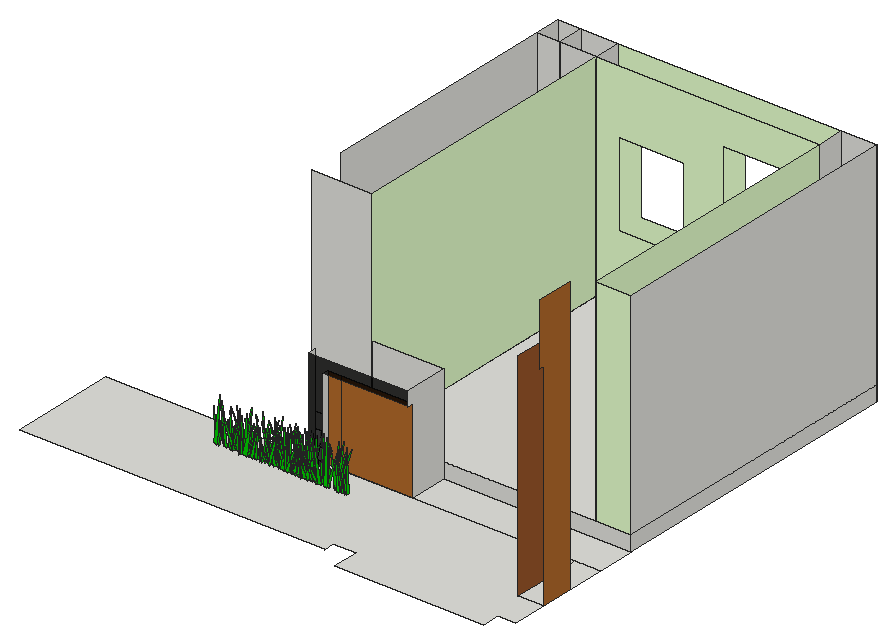
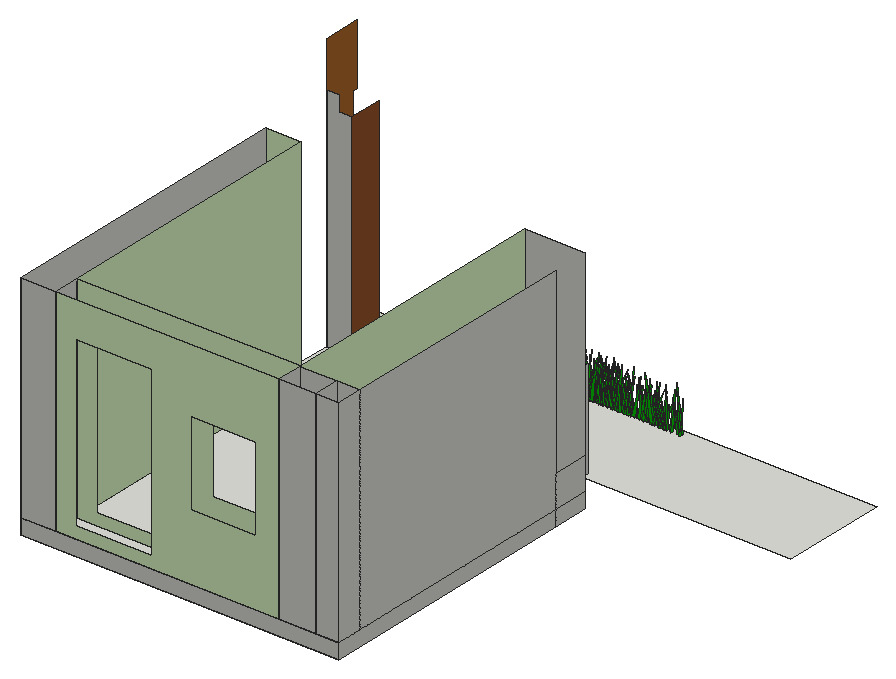
# SketchUp Ruby script. Lengths in inches.
U = 1.inch
M = Sketchup.active_model
def pt(a) = Geom::Point3d.new(a.map { |v| v * U })
def face(e, loops, mat)
  f = e.add_face(loops[0].map { |a| pt(a) })
  loops[1..].each { |l| e.add_face(l.map { |a| pt(a) }).erase! }
  f.material = f.back_material = mat if mat
  f
end
# faces: each face lists its corners as indices into pts; further lists are holes
def faces(e, pts, list, mat = nil) = list.each { |f| face(e, (f[0].is_a?(Array) ? f : [f]).map { |l| l.map { |i| pts[i] } }, mat) }
# xy, xz, yz: faces in a plane at the given z, y or x. An outline is a flat list of corners, or four numbers for a rectangle; further outlines are holes
def ring(l) = l.size == 4 ? [[l[0], l[1]], [l[2], l[1]], [l[2], l[3]], [l[0], l[3]]] : l.each_slice(2).to_a
def flat(e, list, mat, &to3) = list.each { |f| face(e, (f[0].is_a?(Array) ? f : [f]).map { |l| ring(l).map { |u, v| to3.(u, v) } }, mat) }
def xy(e, z, list, mat = nil) = flat(e, list, mat) { |x, y| [x, y, z] }
def xz(e, y, list, mat = nil) = flat(e, list, mat) { |x, z| [x, y, z] }
def yz(e, x, list, mat = nil) = flat(e, list, mat) { |y, z| [x, y, z] }
def lines(e, pts, list) = list.each { |a, b| e.add_line(pt(pts[a]), pt(pts[b])) }
# prism: a flat outline (further loops are holes) pulled along v
def prism(e, loops, v, mat = nil)
  f = face(e, loops, mat); d = Geom::Vector3d.new(v.map { |x| x * U })
  f.pushpull(f.normal.samedirection?(d) ? d.length : -d.length)
end
def box(e, o, s, mat = nil) = prism(e, [[o, [o[0] + s[0], o[1], o[2]], [o[0] + s[0], o[1] + s[1], o[2]], [o[0], o[1] + s[1], o[2]]]], [0, 0, s[2]], mat)
def at(x, y, z, deg = 0) = Geom::Transformation.translation(pt([x, y, z])) * Geom::Transformation.rotation(ORIGIN, Z_AXIS, deg.degrees)
def axes(o, x, y, z) = Geom::Transformation.new([*x, 0, *y, 0, *z, 0, *pt(o).to_a, 1])
def part(name) = M.definitions.add(name)
# library, detail: a bought-in or finely detailed component or shape, given as its bounding box
def library(name, o, s) = part(name).tap { |d| box(d.entities, o, s) }
def detail(e, o, s) = box(e.add_group.entities, o, s)
def put(e, d, t, mat = nil) = e.add_instance(d, t).tap { |i| i.material = mat if mat }
def group(e, t, mat = nil) = e.add_group.tap { |g| g.transformation = t; g.material = mat if mat }.entities
root = M.entities
M.materials.add("[Color F01]1").color = [229, 255, 204]
M.materials.add("[Color G06]").color = [0, 204, 0]
M.materials.add("[Color I07]").color = [0, 0, 0]
M.materials["[Color I07]"].alpha = 0.79
M.materials.add("[Wood Bamboo]").color = [177, 105, 43]
M.materials.add("[Wood Cherry Original]").color = [152, 86, 42]
c1 = part("fur_instance\#9")
p = [[0.8125,0,1.79],[0.67,-0.02,1.48],[0,-0.11,0],[0,0.11,0]]
faces(c1.entities,p,[[0,1,2,3]])
xy(root,-6,[[130.61,2.125,130.61,12.75,121.67,12.5,121.67,8.29,121.48,8.54,2.44,8.54,2.44,50.4375,84.05,50.4375,84.05,47.875,89.3,47.875,89.3,50.4375,185.87,50.4375,185.87,22.6875,196.0625,22.6875,196.0625,9.15,189.03,9.15,189.03,2.125],[185.87,22.6875,195.87,35.6875],[185.87,35.6875,185.87,50.4375,196.01,50.4375,195.87,35.6875],[84.05,47.875,89.3,50.4375],[94.55,50.4375,122.48,65.625],
  [122.48,50.4375,196.01,65.625],[71,65.625,195.87,185.625]])
xy(root,0,[[71,65.625,80,175.4375],[80,65.625,94.55,175.4375],[94.55,65.625,182,175.125],[182,65.625,195.87,185.625],[94.55,175.125,182,185.625],
  [71,175.4375,80,185.625],[80,175.4375,94.55,185.625]])
xz(root,35.6875,[[185.87,-6,185.87,78.0625,191,78.0625,191,84,195.87,84,195.87,-6]])
xz(root,47.875,[[84.05,-6,89.3,-6,89.3,26.81,122.48,26.81,122.48,32.52,84.05,32.52]],"[Color I07]")
xz(root,50.4375,[[89.3,-6,94.55,26.81],[94.55,-6,122.48,26.81]],"[Wood Bamboo]")
xz(root,65.625,[[71,-6,80,0],[80,-6,94.55,0],[94.55,-6,122.48,0],[122.48,-6,195.87,0],[71,0,94.55,84],
  [94.55,0,122.48,32.52]])
xz(root,65.625,[[182,0,195.87,84]],"[Color F01]1")
xz(root,175.125,[[[94.55,0,182,84],[144.35,4.64,174.23,70.2],[103.63,26.05,128.94,58.99]]],"[Color F01]1")
xz(root,175.4375,[[71,0,80,84],[80,0,94.55,84]])
xz(root,185.625,[[71,-6,195.87,0],[71,0,80,84],[80,0,94.55,84],[182,0,195.87,84]])
xz(root,185.625,[[[94.55,0,182,84],[144.35,4.64,174.23,70.2],[103.63,26.05,128.94,58.99]]],"[Color F01]1")
yz(root,71,[[65.625,-6,79.8125,0],[79.8125,-6,185.625,0],[65.625,0,79.8125,12.68],[79.8125,0,175.4375,84],[175.4375,0,185.625,84]])
yz(root,80,[[175.4375,0,185.625,84]])
yz(root,84.05,[[47.875,-6,50.4375,32.52]])
yz(root,89.3,[[47.875,-6,50.4375,26.81]])
yz(root,94.55,[[175.4375,0,185.625,84]])
yz(root,94.55,[[65.625,0,175.125,84],[175.125,0,175.4375,84]],"[Color F01]1")
yz(root,122.48,[[50.4375,-6,65.625,-6,65.625,32.52,47.875,32.52,47.875,26.81,50.4375,26.81]])
yz(root,182,[[175.125,0,185.625,84]])
yz(root,182,[[65.625,0,175.125,84]],"[Color F01]1")
yz(root,185.87,[[22.6875,-6,35.6875,78.0625]],"[Wood Cherry Original]")
yz(root,195.87,[[65.625,-6,185.625,0],[65.625,0,185.625,84]])
yz(root,195.87,[[22.6875,-6,35.6875,-6,35.6875,102,20.8125,102,20.8125,78.0625,22.6875,78.0625]],"[Wood Bamboo]")
put(root,c1,axes([75.34,24.46,4.28],[5.10343,0.12285,3.22807],[-0.02402,-0.7217,3.24002],[-2.33251,0.27623,7.02951]),"[Color G06]")
put(root,c1,axes([99.62,24.86,4.28],[-6.18682,0.07422,0.34005],[0.5595,0.85407,1.325],[0.14833,-0.12594,9.18574]),"[Color G06]")
put(root,c1,axes([93.21,25.05,4.28],[3.0528,-0.63034,1.24282],[-4.3018,-0.44088,-2.08335],[-1.61847,-0.01714,7.88165]),"[Color G06]")
put(root,c1,axes([81.51,24.9,4.28],[1.96052,0.43562,3.15755],[3.76293,-0.24803,-1.28802],[-0.25071,-0.31624,5.35969]),"[Color G06]")
put(root,c1,axes([90.72,24.65,4.28],[-5.23504,-0.16644,2.63846],[-1.62982,0.73337,-1.90895],[1.3729,0.23595,7.79458]),"[Color G06]")
put(root,c1,axes([106.52,24.88,4.28],[-1.70627,-0.75195,2.26774],[-5.55916,0.20005,-1.72315],[-0.68996,0.24771,8.27569]),"[Color G06]")
put(root,c1,axes([105.29,25,4.28],[-4.63412,-0.28911,0.85018],[-1.96778,0.64631,1.28845],[0.86597,-0.0785,7.47741]),"[Color G06]")
put(root,c1,axes([77.09,25.05,4.28],[-0.43919,-0.74626,0.99346],[-5.32471,0.07474,1.19088],[0.85396,0.0822,7.93644]),"[Color G06]")
put(root,c1,axes([93.87,24.78,4.28],[1.03593,0.43975,0.89067],[3.01258,-0.10313,-1.97757],[1.10661,-0.13091,4.54986]),"[Color G06]")
put(root,c1,axes([116.52,24.76,4.28],[-3.63715,-0.14494,0.29928],[-1.05019,0.4816,-1.71614],[-0.1325,0.16148,5.38684]),"[Color G06]")
put(root,c1,axes([84.53,24.5,4.28],[4.87179,0.34836,0.61398],[2.1854,-0.64136,3.06789],[-1.27813,0.23119,7.58585]),"[Color G06]")
put(root,c1,axes([99.4,24.52,4.28],[5.14368,0.17499,2.53292],[0.42709,-0.69653,3.59062],[-2.06508,0.29181,7.05156]),"[Color G06]")
put(root,c1,axes([117.28,25.2,4.28],[3.90904,-0.65856,1.13096],[-4.45698,-0.551,-2.44625],[-1.73542,-0.0683,8.83005]),"[Color G06]")
put(root,c1,axes([90.63,25.0625,4.28],[3.01296,-0.35739,1.87932],[-2.20786,-0.45333,-1.9966],[-1.80976,-0.04195,5.56457]),"[Color G06]")
put(root,c1,axes([65.65,24.8125,4.28],[-1.25759,0.77047,3.12314],[5.7288,0.23173,-1.41438],[1.44073,-0.24892,8.35013]),"[Color G06]")
put(root,c1,axes([94.13,25.15,4.28],[2.44297,-0.59493,0.69898],[-4.20223,-0.34682,-1.10269],[-0.87292,0.0046,7.26457]),"[Color G06]")
put(root,c1,axes([113.01,24.97,4.28],[3.91866,0.45232,1.68058],[3.42442,-0.4981,-2.43574],[0.24373,-0.274,7.20216]),"[Color G06]")
put(root,c1,axes([108.96,24.64,4.28],[-4.78714,0.47855,2.19286],[3.02844,0.69253,-2.59334],[2.1814,0.08875,8.41262]),"[Color G06]")
put(root,c1,axes([103.16,25.03,4.28],[-3.22149,0.07162,0.95824],[0.69679,0.42988,1.54147],[0.43517,-0.1581,4.62547]),"[Color G06]")
put(root,c1,axes([85.16,24.96,4.28],[-3.12966,0.15207,0.38907],[1.12036,0.41998,1.27337],[-0.04366,-0.12408,4.78688]),"[Color G06]")
put(root,c1,axes([80.05,24.79,4.28],[-1.38074,0.43526,1.60713],[2.91328,0.2371,-1.78579],[1.55314,-0.05778,4.77841]),"[Color G06]")
put(root,c1,axes([77.43,24.65,4.28],[0.08241,0.81991,0.71313],[5.76352,0.00299,-1.88339],[1.25764,-0.06745,8.58449]),"[Color G06]")
put(root,c1,axes([106.53,25.01,4.28],[5.52921,0.30513,3.04479],[2.57768,-0.78911,-1.37174],[-1.51458,-0.22908,8.7809]),"[Color G06]")
put(root,c1,axes([95.38,24.99,4.28],[2.88836,0.18057,0.22015],[1.2623,-0.3752,-1.64277],[0.32409,-0.14789,4.43644]),"[Color G06]")
put(root,c1,axes([108.19,25.02,4.28],[0.18644,-0.38744,0.91916],[-2.68202,0.0048,1.44761],[0.95109,0.08948,3.90202]),"[Color G06]")
put(root,c1,axes([75.42,25.11,4.28],[-3.74069,-0.33337,1.23966],[-2.26406,0.53312,1.20854],[1.1302,-0.03541,6.52399]),"[Color G06]")
put(root,c1,axes([103.26,25.14,4.28],[-2.31986,-0.7179,2.75453],[-4.92875,0.39543,2.56652],[2.3682,0.11973,8.0398]),"[Color G06]")
put(root,c1,axes([109.71,24.93,4.28],[3.94342,-0.42779,1.16531],[-3.14625,-0.51072,2.24534],[0.34671,0.23102,7.12156]),"[Color G06]")
put(root,c1,axes([110.07,25.13,4.28],[4.13428,0.14647,3.52348],[1.76209,-0.61378,-1.68746],[-1.88578,-0.25241,6.14791]),"[Color G06]")
put(root,c1,axes([83.16,24.75,4.28],[-3.65968,-0.0806,3.02834],[-1.41288,0.51397,-2.24266],[1.56313,0.27587,5.06299]),"[Color G06]")
put(root,c1,axes([103.8125,25.19,4.28],[-0.43652,-0.61882,0.52237],[-4.30704,0.07109,1.6342],[1.12468,0.03205,6.46104]),"[Color G06]")
put(root,c1,axes([96.16,25.23,4.28],[-0.53636,-0.70646,0.68312],[-4.75082,0.09248,2.6539],[1.81802,0.03323,7.13668]),"[Color G06]")
put(root,c1,axes([77.69,25.1,4.28],[1.03481,-0.40608,0.10722],[-2.82819,-0.13751,1.14346],[0.69783,0.04487,4.47524]),"[Color G06]")
put(root,c1,axes([110.04,24.8125,4.28],[-2.07409,0.24669,0.07508],[1.68594,0.27869,-1.15532],[0.53839,0.07767,3.90711]),"[Color G06]")
put(root,c1,axes([101.35,25.1,4.28],[-1.73258,-0.55974,0.6819],[-3.93374,0.21798,-1.77148],[-0.92011,0.12208,6.2896]),"[Color G06]")
put(root,c1,axes([87.09,25.11,4.28],[-4.50617,0.29239,1.56589],[2.3348,0.58793,2.39698],[0.20762,-0.26556,7.03087]),"[Color G06]")
put(root,c1,axes([93.55,25.09,4.28],[-0.36138,-0.51382,1.32153],[-3.69887,0.02092,-1.32482],[-0.8232,0.13155,5.37263]),"[Color G06]")
put(root,c1,axes([105.22,25.01,4.28],[-2.51703,-0.52895,0.22037],[-3.05345,0.26745,-4.15902],[-2.2554,0.22822,5.3847]),"[Color G06]")
put(root,c1,axes([71.06,25.29,4.28],[-1.84274,-0.71867,0.90946],[-4.99521,0.27004,1.90529],[1.40702,0.01748,7.95531]),"[Color G06]")
put(root,c1,axes([101.06,25.04,4.28],[1.46522,-0.7922,2.854],[-5.32314,-0.04605,4.63628],[2.75409,0.33246,7.44267]),"[Color G06]")
put(root,c1,axes([80.43,25.375,4.28],[1.13466,-0.70996,0.06696],[-4.59461,-0.14553,-3.34579],[-2.1939,-0.0624,7.04159]),"[Color G06]")
put(root,c1,axes([86.57,24.96,4.28],[2.951,0.64433,1.08034],[4.56864,-0.37166,-2.41253],[1.00037,-0.20339,7.83098]),"[Color G06]")
put(root,c1,axes([96.22,24.95,4.28],[0.64897,0.60903,1.74815],[4.33536,-0.03704,-2.11275],[1.28363,-0.18281,6.25185]),"[Color G06]")
put(root,c1,axes([72.8,24.94,4.28],[-0.58311,0.5586,1.24548],[3.54413,0.0103,3.17574],[-2.04461,-0.14145,5.14964]),"[Color G06]")
put(root,c1,axes([78.52,25.07,4.28],[4.27344,0.38949,0.96178],[2.85641,-0.56532,-2.05115],[0.23796,-0.20875,7.34936]),"[Color G06]")
put(root,c1,axes([67.41,24.8,4.28],[4.09785,0.24681,0.79974],[1.52187,-0.55323,2.19427],[-1.05022,0.16135,6.30022]),"[Color G06]")
put(root,c1,axes([97.56,25.03,4.28],[-1.6629,0.38224,0.36635],[2.36872,0.17846,2.62736],[-1.40105,-0.15196,4.00719]),"[Color G06]")
put(root,c1,axes([109.21,24.99,4.28],[2.6719,0.68304,4.21102],[5.02185,-0.48628,1.94339],[-2.59088,-0.23815,8.10954]),"[Color G06]")
put(root,c1,axes([77.76,25.07,4.28],[-0.71443,-0.37443,2.1627],[-2.77276,0.16608,1.25704],[1.27103,0.15185,3.95789]),"[Color G06]")
put(root,c1,axes([75.97,24.83,4.28],[2.26297,0.44488,0.35529],[3.0229,-0.31064,1.67465],[-1.04738,0.06466,5.60095]),"[Color G06]")
put(root,c1,axes([92.95,25.22,4.28],[-5.25093,0.45411,0.49861],[3.03858,0.6434,4.16512],[-1.2179,-0.35262,8.24198]),"[Color G06]")
put(root,c1,axes([71.6875,25.1,4.28],[-0.34441,0.3859,2.05338],[2.90002,0.10688,-1.22087],[1.06588,-0.1661,3.98521]),"[Color G06]")
put(root,c1,axes([81.09,25.23,4.28],[0.52841,-0.57467,1.80389],[-4.13674,-0.11363,-1.45154],[-1.15239,0.14438,6.03775]),"[Color G06]")
put(root,c1,axes([97.25,25.59,4.28],[-5.29054,-0.26219,2.35652],[-0.72253,0.66583,4.88658],[2.34504,-0.38636,6.82205]),"[Color G06]")
put(root,c1,axes([100.86,25.13,4.28],[-2.16589,0.39433,1.17608],[2.92046,0.27579,1.39113],[-0.29491,-0.16491,5.13872]),"[Color G06]")
put(root,c1,axes([97.13,25.47,4.28],[3.86154,-0.28337,0.77524],[-1.54795,-0.48734,-3.24015],[-1.41508,-0.24018,5.6599]),"[Color G06]")
put(root,c1,axes([106.88,25.1,4.28],[4.82769,-0.175,0.06186],[-1.23848,-0.65986,1.46227],[0.20688,0.13347,7.31033]),"[Color G06]")
put(root,c1,axes([113.73,24.82,4.28],[-3.55299,0.42872,0.23933],[2.8143,0.46612,-2.59213],[1.24808,0.16941,6.52635]),"[Color G06]")
put(root,c1,axes([92.21,25.5,4.28],[4.39266,-0.19228,1.10958],[-0.81387,-0.54367,-3.6257],[-1.33797,-0.30057,5.84831]),"[Color G06]")
put(root,c1,axes([97.32,24.93,4.28],[1.66866,0.52368,0.72105],[3.57324,-0.24212,1.7288],[-1.25231,0.00695,5.89362]),"[Color G06]")
put(root,c1,axes([96.08,25.25,4.28],[-1.39254,-0.44701,0.41503],[-3.02265,0.16727,-1.9583],[-1.10299,0.10596,4.84257]),"[Color G06]")
put(root,c1,axes([99.21,25.43,4.28],[-5.79916,-0.05175,2.99276],[0.30319,0.8114,2.92414],[2.01382,-0.27119,8.17793]),"[Color G06]")
put(root,c1,axes([101.58,25.42,4.28],[0.26465,-0.83814,0.9181],[-5.97077,-0.02317,1.41474],[0.9239,0.09035,8.87987]),"[Color G06]")
put(root,c1,axes([88.875,24.96,4.28],[0.61265,0.57685,0.82953],[3.66652,-0.11176,2.87881],[-1.99427,-0.02826,5.54759]),"[Color G06]")
put(root,c1,axes([103.23,25.32,4.28],[1.97884,-0.76286,3.13302],[-5.35719,-0.36051,-2.52551],[-2.37134,0.17784,8.31993]),"[Color G06]")
put(root,c1,axes([95.48,25.34,4.28],[-3.94524,-0.10524,0.90067],[-0.57354,0.53965,1.63193],[0.77706,-0.13603,5.77731]),"[Color G06]")
put(root,c1,axes([101.28,25.23,4.28],[-2.86497,-0.55708,0.2342],[-3.63737,0.35203,-3.20158],[-1.65946,0.19015,6.61322]),"[Color G06]")
put(root,c1,axes([77.7,25.2,4.28],[2.6578,0.34778,1.33581],[2.64887,-0.3522,-1.23893],[-0.05063,-0.16984,5.30458]),"[Color G06]")
put(root,c1,axes([88.71,25.32,4.28],[2.0095,-0.38788,1.4865],[-2.64547,-0.31093,-1.33178],[-1.31449,0.03281,4.95272]),"[Color G06]")
put(root,c1,axes([93.27,25.22,4.28],[-3.728,0.47946,1.58479],[3.58305,0.47521,2.31185],[-0.32907,-0.25746,7.21857]),"[Color G06]")
put(root,c1,axes([113.55,25.12,4.28],[3.701,0.67703,0.92568],[4.73865,-0.46853,-2.95502],[1.22524,-0.23299,8.63247]),"[Color G06]")
put(root,c1,axes([68.82,25.15,4.28],[-3.39639,-0.25699,1.00881],[-1.96018,0.45367,-1.46492],[0.09932,0.16537,5.58645]),"[Color G06]")
put(root,c1,axes([71.73,25.25,4.28],[1.80339,-0.52513,0.97957],[-3.60965,-0.20071,2.48378],[1.25752,0.17694,5.72478]),"[Color G06]")
put(root,c1,axes([97.94,24.96,4.28],[-2.22975,0.61361,1.05459],[4.28149,0.32548,-1.53417],[1.23693,-0.02049,7.21143]),"[Color G06]")
put(root,c1,axes([95.36,25.16,4.28],[-3.04843,-0.28679,1.48008],[-2.25988,0.41162,-1.23496],[0.32136,0.17418,5.35546]),"[Color G06]")
put(root,c1,axes([100.29,24.98,4.28],[-2.5345,0.77322,0.22246],[5.42822,0.34104,1.97491],[-1.14175,-0.09505,8.89549]),"[Color G06]")
put(root,c1,axes([115.49,24.99,4.28],[1.92247,0.6389,1.32637],[4.39262,-0.29293,1.98719],[-1.5763,-0.03708,7.15529]),"[Color G06]")
put(root,c1,axes([79.41,25.02,4.28],[0.24767,0.56277,0.44486],[3.86056,-0.04533,1.78581],[-1.21326,-0.02934,5.77319]),"[Color G06]")
put(root,c1,axes([113.1875,25.19,4.28],[5.12906,-0.4125,2.63009],[-3.28623,-0.71784,1.38212],[-1.02371,0.23763,8.74071]),"[Color G06]")
put(root,c1,axes([91.95,24.98,4.28],[-1.25075,0.64878,0.53364],[4.51034,0.1813,-1.70704],[1.19608,-0.00525,6.99519]),"[Color G06]")
put(root,c1,axes([86.2,25.08,4.28],[-3.83936,0.2109,0.82649],[1.39239,0.53493,-1.23187],[0.80893,0.0802,6.04307]),"[Color G06]")
put(root,c1,axes([103.75,25.4375,4.28],[2.90278,-0.18471,0.99742],[-0.99073,-0.39367,-1.93398],[-1.10378,-0.1324,4.35898]),"[Color G06]")
put(root,c1,axes([113.89,25.31,4.28],[1.07253,-0.4229,0.80971],[-2.89664,-0.11119,1.89924],[1.04898,0.12534,4.41667]),"[Color G06]")
put(root,c1,axes([91.13,25.04,4.28],[-2.63038,0.24841,0.41815],[1.55669,0.34763,-1.85023],[0.91022,0.12334,4.37271]),"[Color G06]")
put(root,c1,axes([94.33,25.53,4.28],[4.5101,-0.4955,1.16478],[-3.32614,-0.63178,-2.10567],[-1.47336,-0.09053,8.3191]),"[Color G06]")
put(root,c1,axes([73.06,25.25,4.28],[-2.71803,0.48242,2.03578],[3.71208,0.36544,1.12253],[0.2109,-0.2149,6.47898]),"[Color G06]")
put(root,c1,axes([93.61,25.04,4.28],[-0.62274,0.65362,0.38062],[4.64165,0.0804,1.10413],[-0.70026,-0.04836,6.98022]),"[Color G06]")
put(root,c1,axes([94.08,25.6,4.28],[4.35442,-0.2361,2.61358],[-0.66734,-0.59641,-3.70561],[-2.3408,-0.26917,5.91828]),"[Color G06]")
put(root,c1,axes([68.83,25.66,4.28],[-4.08111,-0.55124,0.13796],[-3.71674,0.54109,2.764],[1.34956,-0.17679,8.02939]),"[Color G06]")
put(root,c1,axes([96.46,25.0625,4.28],[-0.16308,0.62689,0.55523],[4.18452,0.04038,-2.4925],[1.68478,-0.03962,6.24439]),"[Color G06]")
put(root,c1,axes([95.53,25.5,4.28],[5.24102,0.23519,3.13369],[2.35597,-0.71034,-2.67748],[-1.30006,-0.33915,7.78091]),"[Color G06]")
put(root,c1,axes([106.23,25.4,4.28],[-2.82403,-0.54581,0.03964],[-3.59368,0.35973,-2.88524],[-1.55134,0.16026,6.61151]),"[Color G06]")
put(root,c1,axes([65.4375,25.54,4.28],[-4.12381,-0.25112,1.72545],[-1.44659,0.58493,2.0567],[1.57587,-0.12021,6.40322]),"[Color G06]")
put(root,c1,axes([98.29,25.09,4.28],[-2.98417,0.37885,0.36014],[2.50847,0.40077,-2.00058],[1.07082,0.11693,5.69009]),"[Color G06]")
put(root,c1,axes([79.74,25.11,4.28],[-2.93079,0.37146,0.09531],[2.55893,0.39605,-1.54961],[0.74301,0.10123,5.71284]),"[Color G06]")
put(root,c1,axes([101.4375,25.54,4.28],[4.6377,0.24568,2.29326],[2.23783,-0.60376,-2.67878],[-0.67123,-0.31541,6.91389]),"[Color G06]")
put(root,c1,axes([85.75,25.57,4.28],[-2.95863,-0.19372,0.92818],[-1.06631,0.399,1.9742],[1.08567,-0.13604,4.46843]),"[Color G06]")
put(root,c1,axes([96.6,25.46,4.28],[-2.08211,-0.42678,0.36549],[-3.02517,0.27813,-1.18809],[-0.52435,0.09002,5.40326]),"[Color G06]")
put(root,c1,axes([81.75,25.56,4.28],[0.80713,-0.58654,0.88393],[-4.12403,-0.12831,-1.36906],[-1.01702,0.05482,6.25306]),"[Color G06]")
put(root,c1,axes([69.82,25.05,4.28],[-5.11506,0.39869,0.35172],[2.68356,0.68868,-2.50161],[1.01419,0.18856,8.39319]),"[Color G06]")
put(root,c1,axes([103.01,25.14,4.28],[-2.65967,0.39153,0.27788],[2.62397,0.35798,-1.84049],[1.01626,0.10039,5.47936]),"[Color G06]")
put(root,c1,axes([81.48,25.01,4.28],[3.30883,0.63431,0.23796],[4.24715,-0.44015,2.86086],[-1.63664,0.1402,7.90514]),"[Color G06]")
put(root,c1,axes([77.33,25.37,4.28],[-2.54959,0.71304,1.46147],[4.74796,0.2562,4.14323],[-2.13542,-0.28171,7.46724]),"[Color G06]")
put(root,c1,axes([86.02,25.52,4.28],[4.20566,-0.59849,0.73662],[-4.29785,-0.5699,1.62152],[0.43824,0.15452,8.83331]),"[Color G06]")
put(root,c1,axes([105.2,25.55,4.28],[-2.43711,0.26766,2.90635],[2.55553,0.35188,1.06405],[0.967,-0.25535,4.51276]),"[Color G06]")
put(root,c1,axes([87.31,25.61,4.28],[-1.852,-0.6219,1.968],[-4.30554,0.304,1.98486],[1.7568,0.08942,6.93913]),"[Color G06]")
put(root,c1,axes([107.63,25.64,4.28],[4.92055,-0.0684,3.16351],[0.11121,-0.72182,-2.17912],[-2.1699,-0.19209,7.06201]),"[Color G06]")
put(root,c1,axes([71.7,25.63,4.28],[2.80884,-0.05621,0.58128],[-0.17503,-0.3515,-2.01553],[-0.53209,-0.18111,3.73149]),"[Color G06]")
put(root,c1,axes([98.4,25.39,4.28],[0.57256,0.42343,1.09175],[2.97739,-0.04274,-1.58385],[0.94295,-0.12216,4.33817]),"[Color G06]")
put(root,c1,axes([84.66,25.28,4.28],[0.5833,0.48676,0.03024],[3.35114,-0.07728,-1.48581],[0.97736,-0.02552,5.07647]),"[Color G06]")
put(root,c1,axes([88.95,25.57,4.28],[3.81877,0.04033,2.71385],[0.68352,-0.57298,-1.17024],[-1.70693,-0.13921,5.60288]),"[Color G06]")
put(root,c1,axes([87.48,25.59,4.28],[0.90037,-0.55341,1.5838],[-3.89295,-0.16323,-1.60853],[-1.31069,0.10466,5.86557]),"[Color G06]")
put(root,c1,axes([76.04,25.55,4.28],[-3.06137,0.1856,1.16395],[1.51528,0.40688,1.44924],[0.2864,-0.16877,4.77407]),"[Color G06]")
put(root,c1,axes([101.82,25.3,4.28],[4.48224,0.35966,3.16295],[2.21047,-0.69033,2.02034],[-2.49898,0.03446,7.46023]),"[Color G06]")
put(root,c1,axes([105.76,25.6,4.28],[1.47792,-0.6077,1.21385],[-4.37277,-0.18024,1.52701],[0.7282,0.15104,6.70598]),"[Color G06]")
put(root,c1,axes([112.76,25.32,4.28],[-0.34725,0.72289,1.46207],[5.0582,0.00679,2.2978],[-1.49849,-0.14459,7.41748]),"[Color G06]")
put(root,c1,axes([101.15,25.68,4.28],[-1.13974,-0.6802,1.53614],[-4.78893,0.19023,1.73927],[1.38426,0.09805,7.28187]),"[Color G06]")
put(root,c1,axes([66.56,25.27,4.28],[-0.61164,0.57375,0.23785],[3.94014,0.08807,-1.77163],[1.19578,0.00328,5.95926]),"[Color G06]")
put(root,c1,axes([75.72,25.44,4.28],[-5.13495,-0.19983,2.00068],[-1.65952,0.72157,-1.23518],[1.04473,0.16402,7.87149]),"[Color G06]")
put(root,c1,axes([83.92,25.58,4.28],[-2.81349,-0.61785,1.60807],[-4.54464,0.36578,-1.61709],[-0.36801,0.2065,7.67586]),"[Color G06]")
put(root,c1,axes([73.58,25.67,4.28],[-2.19076,-0.63425,2.21678],[-4.47374,0.3522,1.69969],[1.69499,0.10982,7.35135]),"[Color G06]")
put(root,c1,axes([72.27,25.47,4.28],[3.06364,-0.36996,1.65174],[-2.87353,-0.39872,1.64615],[-0.05662,0.21743,5.82917]),"[Color G06]")
put(root,c1,axes([114.31,25.63,4.28],[-2.83157,-0.04564,0.83676],[-0.16486,0.38887,1.1903],[0.6272,-0.10382,4.0905]),"[Color G06]")
put(root,c1,axes([89.3,25.46,4.28],[4.44288,-0.54368,3.06571],[-4.34042,-0.60976,1.62856],[-0.75456,0.30632,8.68306]),"[Color G06]")
put(root,c1,axes([99.24,25.48,4.28],[3.61572,-0.17807,0.17727],[-1.2658,-0.48754,1.41152],[0.20627,0.12958,5.55456]),"[Color G06]")
put(root,c1,axes([98.91,25.47,4.28],[1.64022,0.52529,1.67959],[3.92361,-0.2083,-1.0752],[0.24212,-0.18298,6.04577]),"[Color G06]")
put(root,c1,axes([106.9,25.62,4.28],[2.91451,-0.60645,1.4263],[-4.44533,-0.38733,1.37185],[0.25202,0.18126,7.70331]),"[Color G06]")
put(root,c1,axes([97.98,25.59,4.28],[3.56215,0.19596,1.05643],[1.54031,-0.48404,-1.28735],[-0.31924,-0.14886,5.57655]),"[Color G06]")
put(root,c1,axes([115.23,25.375,4.28],[-2.50669,0.44779,1.89],[2.97429,0.39084,-1.82596],[1.75069,-0.02284,5.80831]),"[Color G06]")
put(root,c1,axes([100.3,25.71,4.28],[0.32611,-0.73153,1.60563],[-5.23463,-0.07518,-1.55968],[-1.12841,0.13733,7.69928]),"[Color G06]")
put(root,c1,axes([76.47,25.51,4.28],[0.4364,0.38637,2.1448],[2.70199,-0.14785,1.83161],[-1.56066,-0.14794,3.77084]),"[Color G06]")
put(root,c1,axes([105.13,25.58,4.28],[-4.05502,0.55431,2.47172],[4.28967,0.54723,1.62208],[0.36789,-0.27103,8.3304]),"[Color G06]")
put(root,c1,axes([84.83,25.68,4.28],[5.23758,-0.09904,4.17451],[-0.31642,-0.82279,-1.35554],[-2.86457,-0.09019,7.78242]),"[Color G06]")
put(root,c1,axes([90,25.74,4.28],[5.03173,-0.18355,1.03514],[-1.174,-0.6993,-1.49731],[-0.91329,-0.11236,7.62779]),"[Color G06]")
put(root,c1,axes([76.85,25.48,4.28],[2.569,0.7243,2.06263],[5.37023,-0.33759,-1.32249],[0.21067,-0.22671,8.55908]),"[Color G06]")
put(root,c1,axes([65.61,25.73,4.28],[-1.00411,-0.47138,0.9033],[-3.24137,0.1591,1.48882],[1.13393,0.03737,5.05574]),"[Color G06]")
put(root,c1,axes([97.37,25.67,4.28],[-3.3001,0.09766,1.53432],[0.96665,0.45702,1.30245],[0.78103,-0.15297,4.87098]),"[Color G06]")
put(root,c1,axes([92.82,25.32,4.28],[2.95967,0.62931,0.71767],[4.43486,-0.41801,1.25328],[-0.96411,0.00907,7.96812]),"[Color G06]")
put(root,c1,axes([65.61,25.53,4.28],[3.57236,-0.06943,0.54087],[-0.56525,-0.48767,1.1484],[-0.2436,0.11346,5.26701]),"[Color G06]")
put(root,c1,axes([115.39,25.43,4.28],[-3.98203,-0.08086,0.83426],[-0.76059,0.50656,-2.46923],[0.26331,0.24039,5.48394]),"[Color G06]")
put(root,c1,axes([74.57,25.36,4.28],[4.38325,0.19135,1.70782],[0.77569,-0.58444,3.07526],[-1.60842,0.23961,6.13724]),"[Color G06]")
put(root,c1,axes([116.05,25.5,4.28],[-0.9438,0.70058,1.32475],[5.00767,0.1032,1.6995],[-0.97469,-0.14814,7.44875]),"[Color G06]")
put(root,c1,axes([86.01,25.43,4.28],[4.08407,0.34398,1.46091],[2.14469,-0.57526,2.16683],[-1.56227,0.10951,6.79375]),"[Color G06]")
put(root,c1,axes([111.95,25.58,4.28],[-2.74123,0.63448,3.31888],[4.66094,0.45376,-1.3658],[1.97726,-0.19001,7.82078]),"[Color G06]")
put(root,c1,axes([107.28,25.41,4.28],[4.80859,0.2764,1.20639],[1.66706,-0.65732,2.45757],[-1.34215,0.17383,7.37472]),"[Color G06]")
put(root,c1,axes([90.75,25.46,4.28],[-5.20657,0.38017,0.74089],[2.64569,0.72576,-1.24978],[0.82397,0.07193,8.69452]),"[Color G06]")
put(root,c1,axes([98.6,25.48,4.28],[-0.52829,0.66544,0.48699],[4.63627,0.06,1.81674],[-1.17627,-0.06238,6.94196]),"[Color G06]")
put(root,c1,axes([113.15,25.5,4.28],[3.09288,0.28776,0.53086],[1.84309,-0.41605,1.92078],[-0.99378,0.12396,5.21447]),"[Color G06]")
put(root,c1,axes([92.27,25.74,4.28],[5.39934,0.42115,1.10298],[3.10488,-0.74108,-1.44546],[-0.16067,-0.16816,9.13269]),"[Color G06]")
put(root,c1,axes([113.33,25.73,4.28],[1.80625,0.61547,2.08007],[4.5819,-0.20851,-1.80024],[0.65125,-0.24006,6.89655]),"[Color G06]")
put(root,c1,axes([112.46,25.7,4.28],[1.31698,0.4478,0.64792],[3.13811,-0.15998,-1.54654],[0.80781,-0.10856,4.95154]),"[Color G06]")
put(root,c1,axes([102.9,25.48,4.28],[4.81648,0.06346,0.86849],[0.12205,-0.59607,3.49106],[-0.72791,0.31993,6.33204]),"[Color G06]")
put(root,c1,axes([70.53,25.67,4.28],[-3.03313,0.18918,1.02326],[1.14374,0.42453,-1.44334],[1.00059,0.08821,4.75168]),"[Color G06]")
put(root,c1,axes([89.1,25.66,4.28],[-1.44369,0.50999,0.55048],[3.56619,0.2077,-1.21374],[0.891,-0.00498,5.74986]),"[Color G06]")
put(root,c1,axes([72.76,25.74,4.28],[1.09473,0.40816,0.01245],[2.82219,-0.14686,-1.24321],[0.77629,-0.04168,4.50208]),"[Color G06]")
put(root,c1,axes([71.45,25.73,4.28],[1.4606,0.53567,0.45358],[3.73991,-0.18616,-1.64619],[0.92843,-0.09284,5.91764]),"[Color G06]")
put(root,c1,axes([95.46,25.67,4.28],[-3.19381,0.37137,1.66827],[2.31335,0.46796,-2.07397],[1.7283,0.05991,5.85893]),"[Color G06]")
put(root,c1,axes([100.92,25.73,4.28],[2.80939,0.22919,0.55671],[1.43841,-0.37871,1.69619],[-0.87816,0.11291,4.55934]),"[Color G06]")
